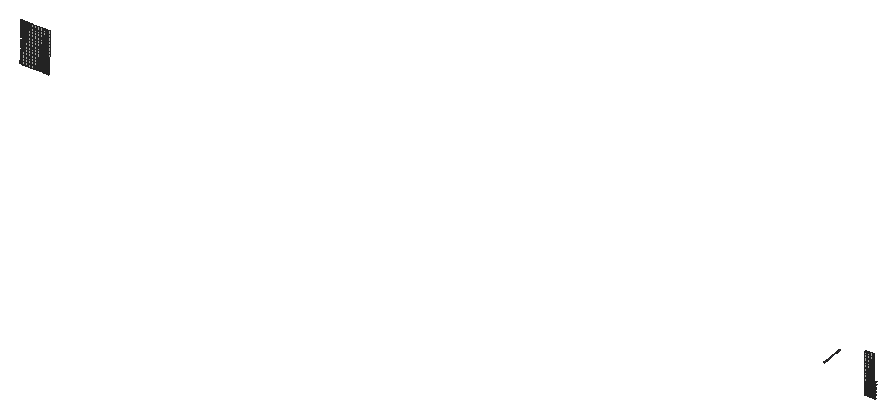
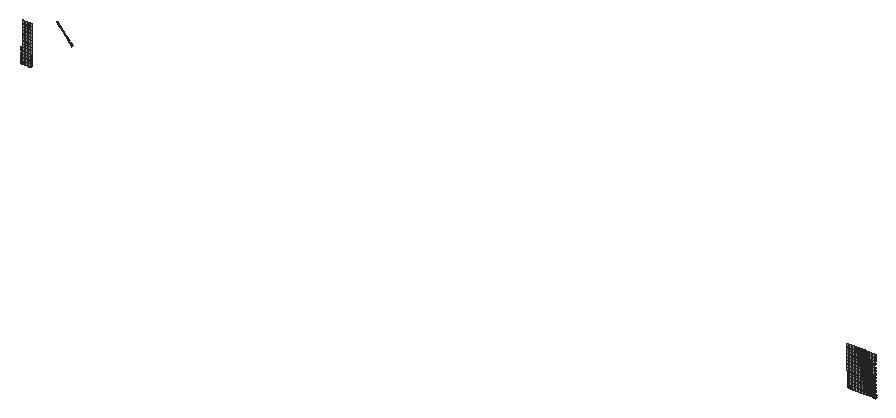
# SketchUp Ruby script. Lengths in inches.
U = 1.inch
M = Sketchup.active_model
def pt(a) = Geom::Point3d.new(a.map { |v| v * U })
def face(e, loops, mat)
  f = e.add_face(loops[0].map { |a| pt(a) })
  loops[1..].each { |l| e.add_face(l.map { |a| pt(a) }).erase! }
  f.material = f.back_material = mat if mat
  f
end
# faces: each face lists its corners as indices into pts; further lists are holes
def faces(e, pts, list, mat = nil) = list.each { |f| face(e, (f[0].is_a?(Array) ? f : [f]).map { |l| l.map { |i| pts[i] } }, mat) }
# xy, xz, yz: faces in a plane at the given z, y or x. An outline is a flat list of corners, or four numbers for a rectangle; further outlines are holes
def ring(l) = l.size == 4 ? [[l[0], l[1]], [l[2], l[1]], [l[2], l[3]], [l[0], l[3]]] : l.each_slice(2).to_a
def flat(e, list, mat, &to3) = list.each { |f| face(e, (f[0].is_a?(Array) ? f : [f]).map { |l| ring(l).map { |u, v| to3.(u, v) } }, mat) }
def xy(e, z, list, mat = nil) = flat(e, list, mat) { |x, y| [x, y, z] }
def xz(e, y, list, mat = nil) = flat(e, list, mat) { |x, z| [x, y, z] }
def yz(e, x, list, mat = nil) = flat(e, list, mat) { |y, z| [x, y, z] }
def lines(e, pts, list) = list.each { |a, b| e.add_line(pt(pts[a]), pt(pts[b])) }
# prism: a flat outline (further loops are holes) pulled along v
def prism(e, loops, v, mat = nil)
  f = face(e, loops, mat); d = Geom::Vector3d.new(v.map { |x| x * U })
  f.pushpull(f.normal.samedirection?(d) ? d.length : -d.length)
end
def box(e, o, s, mat = nil) = prism(e, [[o, [o[0] + s[0], o[1], o[2]], [o[0] + s[0], o[1] + s[1], o[2]], [o[0], o[1] + s[1], o[2]]]], [0, 0, s[2]], mat)
def at(x, y, z, deg = 0) = Geom::Transformation.translation(pt([x, y, z])) * Geom::Transformation.rotation(ORIGIN, Z_AXIS, deg.degrees)
def axes(o, x, y, z) = Geom::Transformation.new([*x, 0, *y, 0, *z, 0, *pt(o).to_a, 1])
def part(name) = M.definitions.add(name)
# library, detail: a bought-in or finely detailed component or shape, given as its bounding box
def library(name, o, s) = part(name).tap { |d| box(d.entities, o, s) }
def detail(e, o, s) = box(e.add_group.entities, o, s)
def put(e, d, t, mat = nil) = e.add_instance(d, t).tap { |i| i.material = mat if mat }
def group(e, t, mat = nil) = e.add_group.tap { |g| g.transformation = t; g.material = mat if mat }.entities
root = M.entities
M.materials.add("[Color M06]").color = [79, 71, 84]
xy(root,265.77,[[1357.11,480.14,1359.42,480.77],[1360.02,480.14,1362.34,480.77],[1362.9375,480.14,1365.25,480.77],[1365.85,480.14,1368.16,480.77],[1368.76,480.14,1371.07,480.77],
  [1371.67,480.14,1373.99,480.77],[1374.58,480.14,1376.9,480.77],[1377.5,480.14,1379.81,480.77],[1380.41,480.14,1382.72,480.77],[1383.32,480.14,1385.63,480.77],
  [2205.72,480.14,2208.03,480.77],[2208.63,480.14,2210.94,480.77],[2211.54,480.14,2213.86,480.77],[2214.46,480.14,2216.77,480.77]])
xy(root,268.09,[[1357.11,480.14,1359.42,480.77],[1360.02,480.14,1362.34,480.77],[1362.9375,480.14,1365.25,480.77],[1365.85,480.14,1368.16,480.77],[1368.76,480.14,1371.07,480.77],
  [1371.67,480.14,1373.99,480.77],[1374.58,480.14,1376.9,480.77],[1377.5,480.14,1379.81,480.77],[1380.41,480.14,1382.72,480.77],[1383.32,480.14,1385.63,480.77],
  [2205.72,480.14,2208.03,480.77],[2208.63,480.14,2210.94,480.77],[2211.54,480.14,2213.86,480.77],[2214.46,480.14,2216.77,480.77]])
xy(root,268.82,[[1357.14,480.14,1359.45,480.77],[1360.05,480.14,1362.37,480.77],[1362.97,480.14,1365.28,480.77],[1365.88,480.14,1368.19,480.77],[1368.79,480.14,1371.1,480.77],
  [1371.7,480.14,1374.01,480.77],[1374.61,480.14,1376.93,480.77],[1377.53,480.14,1379.84,480.77],[1380.4375,480.14,1382.75,480.77],[1383.35,480.14,1385.66,480.77],
  [2205.75,480.14,2208.0625,480.77],[2208.66,480.14,2210.97,480.77],[2211.57,480.14,2213.89,480.77],[2214.49,480.14,2216.8,480.77]])
xy(root,271.13,[[1357.14,480.14,1359.45,480.77],[1360.05,480.14,1362.37,480.77],[1362.97,480.14,1365.28,480.77],[1365.88,480.14,1368.19,480.77],[1368.79,480.14,1371.1,480.77],
  [1371.7,480.14,1374.01,480.77],[1374.61,480.14,1376.93,480.77],[1377.53,480.14,1379.84,480.77],[1380.4375,480.14,1382.75,480.77],[1383.35,480.14,1385.66,480.77],
  [2205.75,480.14,2208.0625,480.77],[2208.66,480.14,2210.97,480.77],[2211.57,480.14,2213.89,480.77],[2214.49,480.14,2216.8,480.77]])
xy(root,271.86,[[1357.17,480.14,1359.48,480.77],[1360.08,480.14,1362.39,480.77],[1362.99,480.14,1365.31,480.77],[1365.91,480.14,1368.22,480.77],[1368.82,480.14,1371.13,480.77],
  [1371.73,480.14,1374.04,480.77],[1374.64,480.14,1376.96,480.77],[1377.55,480.14,1379.87,480.77],[1380.47,480.14,1382.78,480.77],[1383.38,480.14,1385.69,480.77],
  [2205.78,480.14,2208.09,480.77],[2208.69,480.14,2211,480.77],[2211.6,480.14,2213.91,480.77],[2214.51,480.14,2216.83,480.77]])
xy(root,274.17,[[1357.17,480.14,1359.48,480.77],[1360.08,480.14,1362.39,480.77],[1362.99,480.14,1365.31,480.77],[1365.91,480.14,1368.22,480.77],[1368.82,480.14,1371.13,480.77],
  [1371.73,480.14,1374.04,480.77],[1374.64,480.14,1376.96,480.77],[1377.55,480.14,1379.87,480.77],[1380.47,480.14,1382.78,480.77],[1383.38,480.14,1385.69,480.77],
  [2205.78,480.14,2208.09,480.77],[2208.69,480.14,2211,480.77],[2211.6,480.14,2213.91,480.77],[2214.51,480.14,2216.83,480.77]])
xy(root,274.91,[[1357.2,480.14,1359.51,480.77],[1360.11,480.14,1362.42,480.77],[1363.02,480.14,1365.34,480.77],[1365.9375,480.14,1368.25,480.77],[1368.85,480.14,1371.16,480.77],
  [1371.76,480.14,1374.07,480.77],[1374.67,480.14,1376.98,480.77],[1377.58,480.14,1379.9,480.77],[1380.5,480.14,1382.81,480.77],[1383.41,480.14,1385.72,480.77],
  [2205.81,480.14,2208.12,480.77],[2208.72,480.14,2211.03,480.77],[2211.63,480.14,2213.94,480.77],[2214.54,480.14,2216.86,480.77]])
xy(root,277.22,[[1357.2,480.14,1359.51,480.77],[1360.11,480.14,1362.42,480.77],[1363.02,480.14,1365.34,480.77],[1365.9375,480.14,1368.25,480.77],[1368.85,480.14,1371.16,480.77],
  [1371.76,480.14,1374.07,480.77],[1374.67,480.14,1376.98,480.77],[1377.58,480.14,1379.9,480.77],[1380.5,480.14,1382.81,480.77],[1383.41,480.14,1385.72,480.77],
  [2205.81,480.14,2208.12,480.77],[2208.72,480.14,2211.03,480.77],[2211.63,480.14,2213.94,480.77],[2214.54,480.14,2216.86,480.77]])
xy(root,277.95,[[1357.23,480.14,1359.54,480.77],[1360.14,480.14,1362.45,480.77],[1363.05,480.14,1365.36,480.77],[1365.96,480.14,1368.28,480.77],[1368.875,480.14,1371.1875,480.77],
  [1371.79,480.14,1374.1,480.77],[1374.7,480.14,1377.01,480.77],[1377.61,480.14,1379.93,480.77],[1380.52,480.14,1382.84,480.77],[1383.4375,480.14,1385.75,480.77],
  [2205.84,480.14,2208.15,480.77],[2208.75,480.14,2211.06,480.77],[2211.66,480.14,2213.97,480.77],[2214.57,480.14,2216.88,480.77]])
xy(root,280.26,[[1357.23,480.14,1359.54,480.77],[1360.14,480.14,1362.45,480.77],[1363.05,480.14,1365.36,480.77],[1365.96,480.14,1368.28,480.77],[1368.875,480.14,1371.1875,480.77],
  [1371.79,480.14,1374.1,480.77],[1374.7,480.14,1377.01,480.77],[1377.61,480.14,1379.93,480.77],[1380.52,480.14,1382.84,480.77],[1383.4375,480.14,1385.75,480.77],
  [2205.84,480.14,2208.15,480.77],[2208.75,480.14,2211.06,480.77],[2211.66,480.14,2213.97,480.77],[2214.57,480.14,2216.88,480.77]])
xy(root,281,[[1357.26,480.14,1359.57,480.77],[1360.17,480.14,1362.48,480.77],[1363.08,480.14,1365.39,480.77],[1365.99,480.14,1368.31,480.77],[1368.91,480.14,1371.22,480.77],
  [1371.82,480.14,1374.13,480.77],[1374.73,480.14,1377.04,480.77],[1377.64,480.14,1379.95,480.77],[1380.55,480.14,1382.87,480.77],[1383.47,480.14,1385.78,480.77],
  [2205.86,480.14,2208.18,480.77],[2208.78,480.14,2211.09,480.77],[2211.6875,480.14,2214,480.77]])
xy(root,283.31,[[1357.26,480.14,1359.57,480.77],[1360.17,480.14,1362.48,480.77],[1363.08,480.14,1365.39,480.77],[1365.99,480.14,1368.31,480.77],[1368.91,480.14,1371.22,480.77],
  [1371.82,480.14,1374.13,480.77],[1374.73,480.14,1377.04,480.77],[1377.64,480.14,1379.95,480.77],[1380.55,480.14,1382.87,480.77],[1383.47,480.14,1385.78,480.77],
  [2205.86,480.14,2208.18,480.77],[2208.78,480.14,2211.09,480.77],[2211.6875,480.14,2214,480.77]])
xy(root,284.04,[[1357.29,480.14,1359.6,480.77],[1360.2,480.14,1362.51,480.77],[1363.11,480.14,1365.42,480.77],[1366.02,480.14,1368.34,480.77],[1368.93,480.14,1371.25,480.77],
  [1371.85,480.14,1374.16,480.77],[1374.76,480.14,1377.07,480.77],[1377.67,480.14,1379.98,480.77],[1380.58,480.14,1382.9,480.77],[1383.49,480.14,1385.81,480.77],
  [2205.89,480.14,2208.21,480.77],[2208.81,480.14,2211.12,480.77],[2211.72,480.14,2214.03,480.77]])
xy(root,286.35,[[1357.29,480.14,1359.6,480.77],[1360.2,480.14,1362.51,480.77],[1363.11,480.14,1365.42,480.77],[1366.02,480.14,1368.34,480.77],[1368.93,480.14,1371.25,480.77],
  [1371.85,480.14,1374.16,480.77],[1374.76,480.14,1377.07,480.77],[1377.67,480.14,1379.98,480.77],[1380.58,480.14,1382.9,480.77],[1383.49,480.14,1385.81,480.77],
  [2205.89,480.14,2208.21,480.77],[2208.81,480.14,2211.12,480.77],[2211.72,480.14,2214.03,480.77]])
xy(root,287.09,[[1357.32,480.14,1359.63,480.77],[1360.23,480.14,1362.54,480.77],[1363.14,480.14,1365.45,480.77],[1366.05,480.14,1368.36,480.77],[1368.96,480.14,1371.28,480.77],
  [1371.875,480.14,1374.1875,480.77],[1374.79,480.14,1377.1,480.77],[1377.7,480.14,1380.01,480.77],[1380.61,480.14,1382.92,480.77],[1383.52,480.14,1385.84,480.77],
  [2205.92,480.14,2208.24,480.77],[2208.83,480.14,2211.15,480.77],[2211.75,480.14,2214.06,480.77]])
xy(root,289.4,[[1357.32,480.14,1359.63,480.77],[1360.23,480.14,1362.54,480.77],[1363.14,480.14,1365.45,480.77],[1366.05,480.14,1368.36,480.77],[1368.96,480.14,1371.28,480.77],
  [1371.875,480.14,1374.1875,480.77],[1374.79,480.14,1377.1,480.77],[1377.7,480.14,1380.01,480.77],[1380.61,480.14,1382.92,480.77],[1383.52,480.14,1385.84,480.77],
  [2205.92,480.14,2208.24,480.77],[2208.83,480.14,2211.15,480.77],[2211.75,480.14,2214.06,480.77]])
xy(root,290.13,[[1357.34,480.14,1359.66,480.77],[1360.26,480.14,1362.57,480.77],[1363.17,480.14,1365.48,480.77],[1366.08,480.14,1368.39,480.77],[1368.99,480.14,1371.31,480.77],
  [1371.9,480.14,1374.22,480.77],[1374.82,480.14,1377.13,480.77],[1377.73,480.14,1380.04,480.77],[1380.64,480.14,1382.95,480.77],[1383.55,480.14,1385.87,480.77],
  [2205.95,480.14,2208.26,480.77],[2208.86,480.14,2211.18,480.77],[2211.78,480.14,2214.09,480.77]])
xy(root,292.44,[[1357.34,480.14,1359.66,480.77],[1360.26,480.14,1362.57,480.77],[1363.17,480.14,1365.48,480.77],[1366.08,480.14,1368.39,480.77],[1368.99,480.14,1371.31,480.77],
  [1371.9,480.14,1374.22,480.77],[1374.82,480.14,1377.13,480.77],[1377.73,480.14,1380.04,480.77],[1380.64,480.14,1382.95,480.77],[1383.55,480.14,1385.87,480.77],
  [2205.95,480.14,2208.26,480.77],[2208.86,480.14,2211.18,480.77],[2211.78,480.14,2214.09,480.77]])
xy(root,293.18,[[1357.375,480.14,1359.6875,480.77],[1360.29,480.14,1362.6,480.77],[1363.2,480.14,1365.51,480.77],[1366.11,480.14,1368.42,480.77],[1369.02,480.14,1371.33,480.77],
  [1371.93,480.14,1374.25,480.77],[1374.85,480.14,1377.16,480.77],[1377.76,480.14,1380.07,480.77],[1380.67,480.14,1382.98,480.77],[1383.58,480.14,1385.89,480.77],
  [2205.98,480.14,2208.29,480.77],[2208.89,480.14,2211.21,480.77],[2211.8,480.14,2214.12,480.77]])
xy(root,295.49,[[1357.375,480.14,1359.6875,480.77],[1360.29,480.14,1362.6,480.77],[1363.2,480.14,1365.51,480.77],[1366.11,480.14,1368.42,480.77],[1369.02,480.14,1371.33,480.77],
  [1371.93,480.14,1374.25,480.77],[1374.85,480.14,1377.16,480.77],[1377.76,480.14,1380.07,480.77],[1380.67,480.14,1382.98,480.77],[1383.58,480.14,1385.89,480.77],
  [2205.98,480.14,2208.29,480.77],[2208.89,480.14,2211.21,480.77],[2211.8,480.14,2214.12,480.77]])
xy(root,296.22,[[1357.4,480.14,1359.71,480.77],[1360.3125,480.14,1362.625,480.77],[1363.23,480.14,1365.54,480.77],[1366.14,480.14,1368.45,480.77],[1369.05,480.14,1371.36,480.77],
  [1371.96,480.14,1374.28,480.77],[1374.875,480.14,1377.1875,480.77],[1377.79,480.14,1380.1,480.77],[1380.7,480.14,1383.01,480.77],[1383.61,480.14,1385.92,480.77],
  [2206.01,480.14,2208.32,480.77],[2208.92,480.14,2211.23,480.77],[2211.83,480.14,2214.15,480.77]])
xy(root,298.53,[[1357.4,480.14,1359.71,480.77],[1360.3125,480.14,1362.625,480.77],[1363.23,480.14,1365.54,480.77],[1366.14,480.14,1368.45,480.77],[1369.05,480.14,1371.36,480.77],
  [1371.96,480.14,1374.28,480.77],[1374.875,480.14,1377.1875,480.77],[1377.79,480.14,1380.1,480.77],[1380.7,480.14,1383.01,480.77],[1383.61,480.14,1385.92,480.77],
  [2206.01,480.14,2208.32,480.77],[2208.92,480.14,2211.23,480.77],[2211.83,480.14,2214.15,480.77]])
xy(root,299.27,[[1357.43,480.14,1359.74,480.77],[1360.34,480.14,1362.66,480.77],[1363.26,480.14,1365.57,480.77],[1366.17,480.14,1368.48,480.77],[1369.08,480.14,1371.39,480.77],
  [1371.99,480.14,1374.3,480.77],[1374.9,480.14,1377.22,480.77],[1377.82,480.14,1380.13,480.77],[1380.73,480.14,1383.04,480.77],[1383.64,480.14,1385.95,480.77],
  [2206.04,480.14,2208.35,480.77],[2208.95,480.14,2211.26,480.77],[2211.86,480.14,2214.18,480.77]])
xy(root,301.58,[[1357.43,480.14,1359.74,480.77],[1360.34,480.14,1362.66,480.77],[1363.26,480.14,1365.57,480.77],[1366.17,480.14,1368.48,480.77],[1369.08,480.14,1371.39,480.77],
  [1371.99,480.14,1374.3,480.77],[1374.9,480.14,1377.22,480.77],[1377.82,480.14,1380.13,480.77],[1380.73,480.14,1383.04,480.77],[1383.64,480.14,1385.95,480.77],
  [2206.04,480.14,2208.35,480.77],[2208.95,480.14,2211.26,480.77],[2211.86,480.14,2214.18,480.77]])
xy(root,302.31,[[1357.46,480.14,1359.77,480.77],[1360.37,480.14,1362.68,480.77],[1363.28,480.14,1365.6,480.77],[1366.2,480.14,1368.51,480.77],[1369.11,480.14,1371.42,480.77],
  [1372.02,480.14,1374.33,480.77],[1374.93,480.14,1377.25,480.77],[1377.84,480.14,1380.16,480.77],[1380.76,480.14,1383.07,480.77],[1383.67,480.14,1385.98,480.77],
  [2206.07,480.14,2208.38,480.77],[2208.98,480.14,2211.29,480.77],[2211.89,480.14,2214.2,480.77]])
xy(root,304.62,[[1357.46,480.14,1359.77,480.77],[1360.37,480.14,1362.68,480.77],[1363.28,480.14,1365.6,480.77],[1366.2,480.14,1368.51,480.77],[1369.11,480.14,1371.42,480.77],
  [1372.02,480.14,1374.33,480.77],[1374.93,480.14,1377.25,480.77],[1377.84,480.14,1380.16,480.77],[1380.76,480.14,1383.07,480.77],[1383.67,480.14,1385.98,480.77],
  [2206.07,480.14,2208.38,480.77],[2208.98,480.14,2211.29,480.77],[2211.89,480.14,2214.2,480.77]])
xz(root,467.1875,[[2175.5,289.13,2177.93,291.7,2177.47,292.13,2175.05,289.56],[2178.8,292.64,2181.22,295.21,2180.77,295.64,2178.35,293.0625],[2182.1,296.14,2184.52,298.71,2184.07,299.14,2181.65,296.57],[2185.4,299.64,2187.82,302.22,2187.37,302.64,2184.94,300.07],[2188.7,303.15,2191.12,305.72,2190.66,306.15,2188.24,303.58],
  [2188.24,303.58,2190.66,306.15,2190.4375,306.36,2188.02,303.79]],"[Color M06]")
yz(root,1357.43,[[480.14,299.27,480.77,301.58]])
yz(root,1357.46,[[480.14,302.31,480.77,304.62]])
yz(root,1359.42,[[480.14,265.77,480.77,268.09]])
yz(root,1359.45,[[480.14,268.82,480.77,271.13]])
yz(root,1359.48,[[480.14,271.86,480.77,274.17]])
yz(root,1359.51,[[480.14,274.91,480.77,277.22]])
yz(root,1359.54,[[480.14,277.95,480.77,280.26]])
yz(root,1359.57,[[480.14,281,480.77,283.31]])
yz(root,1359.6,[[480.14,284.04,480.77,286.35]])
yz(root,1359.63,[[480.14,287.09,480.77,289.4]])
yz(root,1359.66,[[480.14,290.13,480.77,292.44]])
yz(root,1359.6875,[[480.14,293.18,480.77,295.49]])
yz(root,1359.71,[[480.14,296.22,480.77,298.53]])
yz(root,1359.74,[[480.14,299.27,480.77,301.58]])
yz(root,1359.77,[[480.14,302.31,480.77,304.62]])
yz(root,1360.02,[[480.14,265.77,480.77,268.09]])
yz(root,1360.05,[[480.14,268.82,480.77,271.13]])
yz(root,1360.08,[[480.14,271.86,480.77,274.17]])
yz(root,1360.11,[[480.14,274.91,480.77,277.22]])
yz(root,1360.14,[[480.14,277.95,480.77,280.26]])
yz(root,1360.17,[[480.14,281,480.77,283.31]])
yz(root,1360.2,[[480.14,284.04,480.77,286.35]])
yz(root,1360.23,[[480.14,287.09,480.77,289.4]])
yz(root,1360.26,[[480.14,290.13,480.77,292.44]])
yz(root,1360.29,[[480.14,293.18,480.77,295.49]])
yz(root,1360.3125,[[480.14,296.22,480.77,298.53]])
yz(root,1360.34,[[480.14,299.27,480.77,301.58]])
yz(root,1360.37,[[480.14,302.31,480.77,304.62]])
yz(root,1362.34,[[480.14,265.77,480.77,268.09]])
yz(root,1362.37,[[480.14,268.82,480.77,271.13]])
yz(root,1362.39,[[480.14,271.86,480.77,274.17]])
yz(root,1362.42,[[480.14,274.91,480.77,277.22]])
yz(root,1362.45,[[480.14,277.95,480.77,280.26]])
yz(root,1362.48,[[480.14,281,480.77,283.31]])
yz(root,1362.51,[[480.14,284.04,480.77,286.35]])
yz(root,1362.54,[[480.14,287.09,480.77,289.4]])
yz(root,1362.57,[[480.14,290.13,480.77,292.44]])
yz(root,1362.6,[[480.14,293.18,480.77,295.49]])
yz(root,1362.625,[[480.14,296.22,480.77,298.53]])
yz(root,1362.66,[[480.14,299.27,480.77,301.58]])
yz(root,1362.68,[[480.14,302.31,480.77,304.62]])
yz(root,1362.9375,[[480.14,265.77,480.77,268.09]])
yz(root,1362.97,[[480.14,268.82,480.77,271.13]])
yz(root,1362.99,[[480.14,271.86,480.77,274.17]])
yz(root,1363.02,[[480.14,274.91,480.77,277.22]])
yz(root,1363.05,[[480.14,277.95,480.77,280.26]])
yz(root,1363.08,[[480.14,281,480.77,283.31]])
yz(root,1363.11,[[480.14,284.04,480.77,286.35]])
yz(root,1363.14,[[480.14,287.09,480.77,289.4]])
yz(root,1363.17,[[480.14,290.13,480.77,292.44]])
yz(root,1363.2,[[480.14,293.18,480.77,295.49]])
yz(root,1363.23,[[480.14,296.22,480.77,298.53]])
yz(root,1363.26,[[480.14,299.27,480.77,301.58]])
yz(root,1363.28,[[480.14,302.31,480.77,304.62]])
yz(root,1365.25,[[480.14,265.77,480.77,268.09]])
yz(root,1365.28,[[480.14,268.82,480.77,271.13]])
yz(root,1365.31,[[480.14,271.86,480.77,274.17]])
yz(root,1365.34,[[480.14,274.91,480.77,277.22]])
yz(root,1365.36,[[480.14,277.95,480.77,280.26]])
yz(root,1365.39,[[480.14,281,480.77,283.31]])
yz(root,1365.42,[[480.14,284.04,480.77,286.35]])
yz(root,1365.45,[[480.14,287.09,480.77,289.4]])
yz(root,1365.48,[[480.14,290.13,480.77,292.44]])
yz(root,1365.51,[[480.14,293.18,480.77,295.49]])
yz(root,1365.54,[[480.14,296.22,480.77,298.53]])
yz(root,1365.57,[[480.14,299.27,480.77,301.58]])
yz(root,1365.6,[[480.14,302.31,480.77,304.62]])
yz(root,1365.85,[[480.14,265.77,480.77,268.09]])
yz(root,1365.88,[[480.14,268.82,480.77,271.13]])
yz(root,1365.91,[[480.14,271.86,480.77,274.17]])
yz(root,1365.9375,[[480.14,274.91,480.77,277.22]])
yz(root,1365.96,[[480.14,277.95,480.77,280.26]])
yz(root,1365.99,[[480.14,281,480.77,283.31]])
yz(root,1366.02,[[480.14,284.04,480.77,286.35]])
yz(root,1366.05,[[480.14,287.09,480.77,289.4]])
yz(root,1366.08,[[480.14,290.13,480.77,292.44]])
yz(root,1366.11,[[480.14,293.18,480.77,295.49]])
yz(root,1366.14,[[480.14,296.22,480.77,298.53]])
yz(root,1366.17,[[480.14,299.27,480.77,301.58]])
yz(root,1366.2,[[480.14,302.31,480.77,304.62]])
yz(root,1368.16,[[480.14,265.77,480.77,268.09]])
yz(root,1368.19,[[480.14,268.82,480.77,271.13]])
yz(root,1368.22,[[480.14,271.86,480.77,274.17]])
yz(root,1368.25,[[480.14,274.91,480.77,277.22]])
yz(root,1368.28,[[480.14,277.95,480.77,280.26]])
yz(root,1368.31,[[480.14,281,480.77,283.31]])
yz(root,1368.34,[[480.14,284.04,480.77,286.35]])
yz(root,1368.36,[[480.14,287.09,480.77,289.4]])
yz(root,1368.39,[[480.14,290.13,480.77,292.44]])
yz(root,1368.42,[[480.14,293.18,480.77,295.49]])
yz(root,1368.45,[[480.14,296.22,480.77,298.53]])
yz(root,1368.48,[[480.14,299.27,480.77,301.58]])
yz(root,1368.51,[[480.14,302.31,480.77,304.62]])
yz(root,1368.76,[[480.14,265.77,480.77,268.09]])
yz(root,1368.79,[[480.14,268.82,480.77,271.13]])
yz(root,1368.82,[[480.14,271.86,480.77,274.17]])
yz(root,1368.85,[[480.14,274.91,480.77,277.22]])
yz(root,1368.875,[[480.14,277.95,480.77,280.26]])
yz(root,1368.91,[[480.14,281,480.77,283.31]])
yz(root,1368.93,[[480.14,284.04,480.77,286.35]])
yz(root,1368.96,[[480.14,287.09,480.77,289.4]])
yz(root,1368.99,[[480.14,290.13,480.77,292.44]])
yz(root,1369.02,[[480.14,293.18,480.77,295.49]])
yz(root,1369.05,[[480.14,296.22,480.77,298.53]])
yz(root,1369.08,[[480.14,299.27,480.77,301.58]])
yz(root,1369.11,[[480.14,302.31,480.77,304.62]])
yz(root,1371.07,[[480.14,265.77,480.77,268.09]])
yz(root,1371.1,[[480.14,268.82,480.77,271.13]])
yz(root,1371.13,[[480.14,271.86,480.77,274.17]])
yz(root,1371.16,[[480.14,274.91,480.77,277.22]])
yz(root,1371.1875,[[480.14,277.95,480.77,280.26]])
yz(root,1371.22,[[480.14,281,480.77,283.31]])
yz(root,1371.25,[[480.14,284.04,480.77,286.35]])
yz(root,1371.28,[[480.14,287.09,480.77,289.4]])
yz(root,1371.31,[[480.14,290.13,480.77,292.44]])
yz(root,1371.33,[[480.14,293.18,480.77,295.49]])
yz(root,1371.36,[[480.14,296.22,480.77,298.53]])
yz(root,1371.39,[[480.14,299.27,480.77,301.58]])
yz(root,1371.42,[[480.14,302.31,480.77,304.62]])
yz(root,1371.67,[[480.14,265.77,480.77,268.09]])
yz(root,1371.7,[[480.14,268.82,480.77,271.13]])
yz(root,1371.73,[[480.14,271.86,480.77,274.17]])
yz(root,1371.76,[[480.14,274.91,480.77,277.22]])
yz(root,1371.79,[[480.14,277.95,480.77,280.26]])
yz(root,1371.82,[[480.14,281,480.77,283.31]])
yz(root,1371.85,[[480.14,284.04,480.77,286.35]])
yz(root,1371.875,[[480.14,287.09,480.77,289.4]])
yz(root,1371.9,[[480.14,290.13,480.77,292.44]])
yz(root,1371.93,[[480.14,293.18,480.77,295.49]])
yz(root,1371.96,[[480.14,296.22,480.77,298.53]])
yz(root,1371.99,[[480.14,299.27,480.77,301.58]])
yz(root,1372.02,[[480.14,302.31,480.77,304.62]])
yz(root,1373.99,[[480.14,265.77,480.77,268.09]])
yz(root,1374.01,[[480.14,268.82,480.77,271.13]])
yz(root,1374.04,[[480.14,271.86,480.77,274.17]])
yz(root,1374.07,[[480.14,274.91,480.77,277.22]])
yz(root,1374.1,[[480.14,277.95,480.77,280.26]])
yz(root,1374.13,[[480.14,281,480.77,283.31]])
yz(root,1374.16,[[480.14,284.04,480.77,286.35]])
yz(root,1374.1875,[[480.14,287.09,480.77,289.4]])
yz(root,1374.22,[[480.14,290.13,480.77,292.44]])
yz(root,1374.25,[[480.14,293.18,480.77,295.49]])
yz(root,1374.28,[[480.14,296.22,480.77,298.53]])
yz(root,1374.3,[[480.14,299.27,480.77,301.58]])
yz(root,1374.33,[[480.14,302.31,480.77,304.62]])
yz(root,1374.58,[[480.14,265.77,480.77,268.09]])
yz(root,1374.61,[[480.14,268.82,480.77,271.13]])
yz(root,1374.64,[[480.14,271.86,480.77,274.17]])
yz(root,1374.67,[[480.14,274.91,480.77,277.22]])
yz(root,1374.7,[[480.14,277.95,480.77,280.26]])
yz(root,1374.73,[[480.14,281,480.77,283.31]])
yz(root,1374.76,[[480.14,284.04,480.77,286.35]])
yz(root,1374.79,[[480.14,287.09,480.77,289.4]])
yz(root,1374.82,[[480.14,290.13,480.77,292.44]])
yz(root,1374.85,[[480.14,293.18,480.77,295.49]])
yz(root,1374.875,[[480.14,296.22,480.77,298.53]])
yz(root,1374.9,[[480.14,299.27,480.77,301.58]])
yz(root,1374.93,[[480.14,302.31,480.77,304.62]])
yz(root,1376.9,[[480.14,265.77,480.77,268.09]])
yz(root,1376.93,[[480.14,268.82,480.77,271.13]])
yz(root,1376.96,[[480.14,271.86,480.77,274.17]])
yz(root,1376.98,[[480.14,274.91,480.77,277.22]])
yz(root,1377.01,[[480.14,277.95,480.77,280.26]])
yz(root,1377.04,[[480.14,281,480.77,283.31]])
yz(root,1377.07,[[480.14,284.04,480.77,286.35]])
yz(root,1377.1,[[480.14,287.09,480.77,289.4]])
yz(root,1377.13,[[480.14,290.13,480.77,292.44]])
yz(root,1377.16,[[480.14,293.18,480.77,295.49]])
yz(root,1377.1875,[[480.14,296.22,480.77,298.53]])
yz(root,1377.22,[[480.14,299.27,480.77,301.58]])
yz(root,1377.25,[[480.14,302.31,480.77,304.62]])
yz(root,1377.5,[[480.14,265.77,480.77,268.09]])
yz(root,1377.53,[[480.14,268.82,480.77,271.13]])
yz(root,1377.55,[[480.14,271.86,480.77,274.17]])
yz(root,1377.58,[[480.14,274.91,480.77,277.22]])
yz(root,1377.61,[[480.14,277.95,480.77,280.26]])
yz(root,1377.64,[[480.14,281,480.77,283.31]])
yz(root,1377.67,[[480.14,284.04,480.77,286.35]])
yz(root,1377.7,[[480.14,287.09,480.77,289.4]])
yz(root,1377.73,[[480.14,290.13,480.77,292.44]])
yz(root,1377.76,[[480.14,293.18,480.77,295.49]])
yz(root,1377.79,[[480.14,296.22,480.77,298.53]])
yz(root,1377.82,[[480.14,299.27,480.77,301.58]])
yz(root,1377.84,[[480.14,302.31,480.77,304.62]])
yz(root,1379.81,[[480.14,265.77,480.77,268.09]])
yz(root,1379.84,[[480.14,268.82,480.77,271.13]])
yz(root,1379.87,[[480.14,271.86,480.77,274.17]])
yz(root,1379.9,[[480.14,274.91,480.77,277.22]])
yz(root,1379.93,[[480.14,277.95,480.77,280.26]])
yz(root,1379.95,[[480.14,281,480.77,283.31]])
yz(root,1379.98,[[480.14,284.04,480.77,286.35]])
yz(root,1380.01,[[480.14,287.09,480.77,289.4]])
yz(root,1380.04,[[480.14,290.13,480.77,292.44]])
yz(root,1380.07,[[480.14,293.18,480.77,295.49]])
yz(root,1380.1,[[480.14,296.22,480.77,298.53]])
yz(root,1380.13,[[480.14,299.27,480.77,301.58]])
yz(root,1380.16,[[480.14,302.31,480.77,304.62]])
yz(root,1380.41,[[480.14,265.77,480.77,268.09]])
yz(root,1380.4375,[[480.14,268.82,480.77,271.13]])
yz(root,1380.47,[[480.14,271.86,480.77,274.17]])
yz(root,1380.5,[[480.14,274.91,480.77,277.22]])
yz(root,1380.52,[[480.14,277.95,480.77,280.26]])
yz(root,1380.55,[[480.14,281,480.77,283.31]])
yz(root,1380.58,[[480.14,284.04,480.77,286.35]])
yz(root,1380.61,[[480.14,287.09,480.77,289.4]])
yz(root,1380.64,[[480.14,290.13,480.77,292.44]])
yz(root,1380.67,[[480.14,293.18,480.77,295.49]])
yz(root,1380.7,[[480.14,296.22,480.77,298.53]])
yz(root,1380.73,[[480.14,299.27,480.77,301.58]])
yz(root,1380.76,[[480.14,302.31,480.77,304.62]])
yz(root,1382.72,[[480.14,265.77,480.77,268.09]])
yz(root,1382.75,[[480.14,268.82,480.77,271.13]])
yz(root,1382.78,[[480.14,271.86,480.77,274.17]])
yz(root,1382.81,[[480.14,274.91,480.77,277.22]])
yz(root,1382.84,[[480.14,277.95,480.77,280.26]])
yz(root,1382.87,[[480.14,281,480.77,283.31]])
yz(root,1382.9,[[480.14,284.04,480.77,286.35]])
yz(root,1382.92,[[480.14,287.09,480.77,289.4]])
yz(root,1382.95,[[480.14,290.13,480.77,292.44]])
yz(root,1382.98,[[480.14,293.18,480.77,295.49]])
yz(root,1383.01,[[480.14,296.22,480.77,298.53]])
yz(root,1383.04,[[480.14,299.27,480.77,301.58]])
yz(root,1383.07,[[480.14,302.31,480.77,304.62]])
yz(root,1383.32,[[480.14,265.77,480.77,268.09]])
yz(root,1383.35,[[480.14,268.82,480.77,271.13]])
yz(root,1383.38,[[480.14,271.86,480.77,274.17]])
yz(root,1383.41,[[480.14,274.91,480.77,277.22]])
yz(root,1383.4375,[[480.14,277.95,480.77,280.26]])
yz(root,1383.47,[[480.14,281,480.77,283.31]])
yz(root,1383.49,[[480.14,284.04,480.77,286.35]])
yz(root,1383.52,[[480.14,287.09,480.77,289.4]])
yz(root,1383.55,[[480.14,290.13,480.77,292.44]])
yz(root,1383.58,[[480.14,293.18,480.77,295.49]])
yz(root,1383.61,[[480.14,296.22,480.77,298.53]])
yz(root,1383.64,[[480.14,299.27,480.77,301.58]])
yz(root,1383.67,[[480.14,302.31,480.77,304.62]])
yz(root,1385.63,[[480.14,265.77,480.77,268.09]])
yz(root,1385.66,[[480.14,268.82,480.77,271.13]])
yz(root,1385.69,[[480.14,271.86,480.77,274.17]])
yz(root,1385.72,[[480.14,274.91,480.77,277.22]])
yz(root,1385.75,[[480.14,277.95,480.77,280.26]])
yz(root,1385.78,[[480.14,281,480.77,283.31]])
yz(root,1385.81,[[480.14,284.04,480.77,286.35]])
yz(root,1385.84,[[480.14,287.09,480.77,289.4]])
yz(root,1385.87,[[480.14,290.13,480.77,292.44]])
yz(root,1385.89,[[480.14,293.18,480.77,295.49]])
yz(root,1385.92,[[480.14,296.22,480.77,298.53]])
yz(root,1385.95,[[480.14,299.27,480.77,301.58]])
yz(root,1385.98,[[480.14,302.31,480.77,304.62]])
yz(root,2205.72,[[480.14,265.77,480.77,268.09]])
yz(root,2205.75,[[480.14,268.82,480.77,271.13]])
yz(root,2205.78,[[480.14,271.86,480.77,274.17]])
yz(root,2205.81,[[480.14,274.91,480.77,277.22]])
yz(root,2205.84,[[480.14,277.95,480.77,280.26]])
yz(root,2205.86,[[480.14,281,480.77,283.31]])
yz(root,2205.89,[[480.14,284.04,480.77,286.35]])
yz(root,2205.92,[[480.14,287.09,480.77,289.4]])
yz(root,2205.95,[[480.14,290.13,480.77,292.44]])
yz(root,2205.98,[[480.14,293.18,480.77,295.49]])
yz(root,2206.01,[[480.14,296.22,480.77,298.53]])
yz(root,2206.04,[[480.14,299.27,480.77,301.58]])
yz(root,2206.07,[[480.14,302.31,480.77,304.62]])
yz(root,2208.03,[[480.14,265.77,480.77,268.09]])
yz(root,2208.0625,[[480.14,268.82,480.77,271.13]])
yz(root,2208.09,[[480.14,271.86,480.77,274.17]])
yz(root,2208.12,[[480.14,274.91,480.77,277.22]])
yz(root,2208.15,[[480.14,277.95,480.77,280.26]])
yz(root,2208.18,[[480.14,281,480.77,283.31]])
yz(root,2208.21,[[480.14,284.04,480.77,286.35]])
yz(root,2208.24,[[480.14,287.09,480.77,289.4]])
yz(root,2208.26,[[480.14,290.13,480.77,292.44]])
yz(root,2208.29,[[480.14,293.18,480.77,295.49]])
yz(root,2208.32,[[480.14,296.22,480.77,298.53]])
yz(root,2208.35,[[480.14,299.27,480.77,301.58]])
yz(root,2208.38,[[480.14,302.31,480.77,304.62]])
yz(root,2208.63,[[480.14,265.77,480.77,268.09]])
yz(root,2208.66,[[480.14,268.82,480.77,271.13]])
yz(root,2208.69,[[480.14,271.86,480.77,274.17]])
yz(root,2208.72,[[480.14,274.91,480.77,277.22]])
yz(root,2208.75,[[480.14,277.95,480.77,280.26]])
yz(root,2208.78,[[480.14,281,480.77,283.31]])
yz(root,2208.81,[[480.14,284.04,480.77,286.35]])
yz(root,2208.83,[[480.14,287.09,480.77,289.4]])
yz(root,2208.86,[[480.14,290.13,480.77,292.44]])
yz(root,2208.89,[[480.14,293.18,480.77,295.49]])
yz(root,2208.92,[[480.14,296.22,480.77,298.53]])
yz(root,2208.95,[[480.14,299.27,480.77,301.58]])
yz(root,2208.98,[[480.14,302.31,480.77,304.62]])
yz(root,2210.94,[[480.14,265.77,480.77,268.09]])
yz(root,2210.97,[[480.14,268.82,480.77,271.13]])
yz(root,2211,[[480.14,271.86,480.77,274.17]])
yz(root,2211.03,[[480.14,274.91,480.77,277.22]])
yz(root,2211.06,[[480.14,277.95,480.77,280.26]])
yz(root,2211.09,[[480.14,281,480.77,283.31]])
yz(root,2211.12,[[480.14,284.04,480.77,286.35]])
yz(root,2211.15,[[480.14,287.09,480.77,289.4]])
yz(root,2211.18,[[480.14,290.13,480.77,292.44]])
yz(root,2211.21,[[480.14,293.18,480.77,295.49]])
yz(root,2211.23,[[480.14,296.22,480.77,298.53]])
yz(root,2211.26,[[480.14,299.27,480.77,301.58]])
yz(root,2211.29,[[480.14,302.31,480.77,304.62]])
yz(root,2211.54,[[480.14,265.77,480.77,268.09]])
yz(root,2211.57,[[480.14,268.82,480.77,271.13]])
yz(root,2211.6,[[480.14,271.86,480.77,274.17]])
yz(root,2211.63,[[480.14,274.91,480.77,277.22]])
yz(root,2211.66,[[480.14,277.95,480.77,280.26]])
yz(root,2211.6875,[[480.14,281,480.77,283.31]])
yz(root,2211.72,[[480.14,284.04,480.77,286.35]])
yz(root,2211.75,[[480.14,287.09,480.77,289.4]])
yz(root,2211.78,[[480.14,290.13,480.77,292.44]])
yz(root,2211.8,[[480.14,293.18,480.77,295.49]])
yz(root,2211.83,[[480.14,296.22,480.77,298.53]])
yz(root,2211.86,[[480.14,299.27,480.77,301.58]])
yz(root,2211.89,[[480.14,302.31,480.77,304.62]])
yz(root,2213.86,[[480.14,265.77,480.77,268.09]])
yz(root,2213.89,[[480.14,268.82,480.77,271.13]])
yz(root,2213.91,[[480.14,271.86,480.77,274.17]])
yz(root,2213.94,[[480.14,274.91,480.77,277.22]])
yz(root,2213.97,[[480.14,277.95,480.77,280.26]])
yz(root,2214,[[480.14,281,480.77,283.31]])
yz(root,2214.03,[[480.14,284.04,480.77,286.35]])
yz(root,2214.06,[[480.14,287.09,480.77,289.4]])
yz(root,2214.09,[[480.14,290.13,480.77,292.44]])
yz(root,2214.12,[[480.14,293.18,480.77,295.49]])
yz(root,2214.15,[[480.14,296.22,480.77,298.53]])
yz(root,2214.18,[[480.14,299.27,480.77,301.58]])
yz(root,2214.2,[[480.14,302.31,480.77,304.62]])
yz(root,2214.46,[[480.14,265.77,480.77,268.09]])
yz(root,2214.49,[[480.14,268.82,480.77,271.13]])
yz(root,2214.51,[[480.14,271.86,480.77,274.17]])
yz(root,2214.54,[[480.14,274.91,480.77,277.22]])
yz(root,2214.57,[[480.14,277.95,480.77,280.26]])
yz(root,2214.6,[[480.14,281,480.77,283.31]])
yz(root,2214.63,[[480.14,284.04,480.77,286.35]])
yz(root,2214.66,[[480.14,287.09,480.77,289.4]])
yz(root,2214.6875,[[480.14,290.13,480.77,292.44]])
yz(root,2214.72,[[480.14,293.18,480.77,295.49]])
yz(root,2214.75,[[480.14,296.22,480.77,298.53]])
yz(root,2214.78,[[480.14,299.27,480.77,301.58]])
yz(root,2214.8,[[480.14,302.31,480.77,304.62]])
